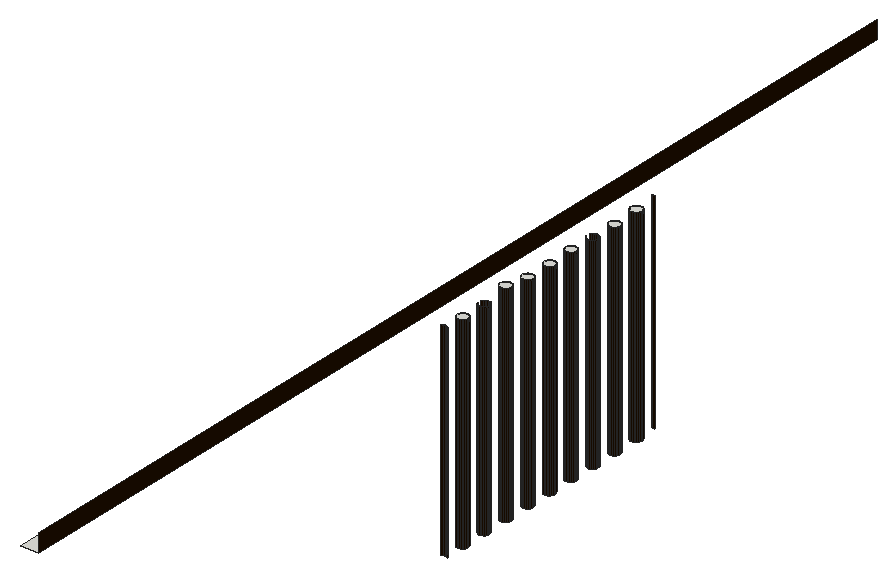
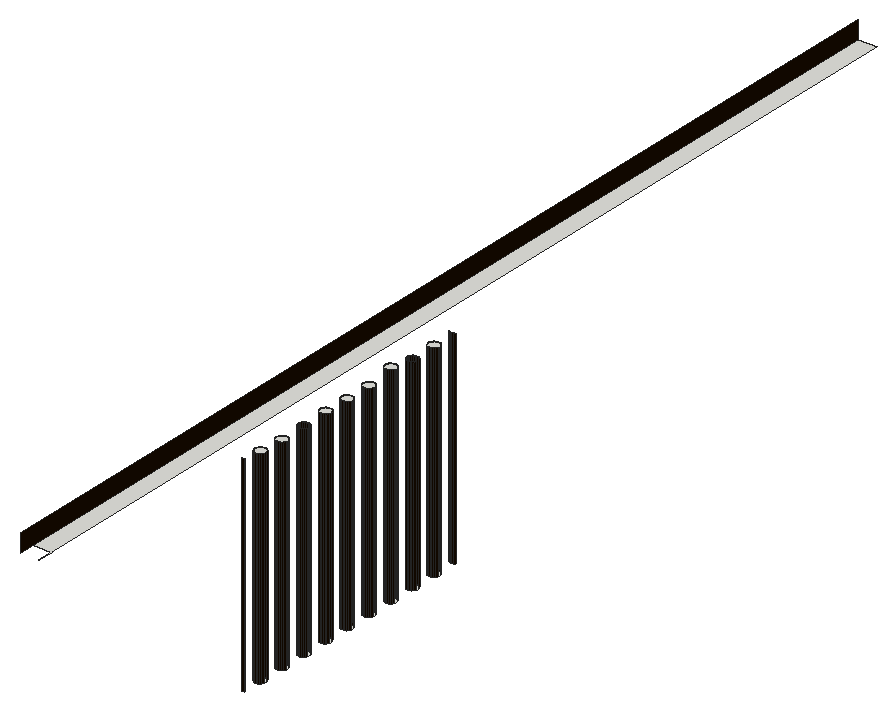
# SketchUp Ruby script. Lengths in inches.
U = 1.inch
M = Sketchup.active_model
def pt(a) = Geom::Point3d.new(a.map { |v| v * U })
def face(e, loops, mat)
  f = e.add_face(loops[0].map { |a| pt(a) })
  loops[1..].each { |l| e.add_face(l.map { |a| pt(a) }).erase! }
  f.material = f.back_material = mat if mat
  f
end
# faces: each face lists its corners as indices into pts; further lists are holes
def faces(e, pts, list, mat = nil) = list.each { |f| face(e, (f[0].is_a?(Array) ? f : [f]).map { |l| l.map { |i| pts[i] } }, mat) }
# xy, xz, yz: faces in a plane at the given z, y or x. An outline is a flat list of corners, or four numbers for a rectangle; further outlines are holes
def ring(l) = l.size == 4 ? [[l[0], l[1]], [l[2], l[1]], [l[2], l[3]], [l[0], l[3]]] : l.each_slice(2).to_a
def flat(e, list, mat, &to3) = list.each { |f| face(e, (f[0].is_a?(Array) ? f : [f]).map { |l| ring(l).map { |u, v| to3.(u, v) } }, mat) }
def xy(e, z, list, mat = nil) = flat(e, list, mat) { |x, y| [x, y, z] }
def xz(e, y, list, mat = nil) = flat(e, list, mat) { |x, z| [x, y, z] }
def yz(e, x, list, mat = nil) = flat(e, list, mat) { |y, z| [x, y, z] }
def lines(e, pts, list) = list.each { |a, b| e.add_line(pt(pts[a]), pt(pts[b])) }
# prism: a flat outline (further loops are holes) pulled along v
def prism(e, loops, v, mat = nil)
  f = face(e, loops, mat); d = Geom::Vector3d.new(v.map { |x| x * U })
  f.pushpull(f.normal.samedirection?(d) ? d.length : -d.length)
end
def box(e, o, s, mat = nil) = prism(e, [[o, [o[0] + s[0], o[1], o[2]], [o[0] + s[0], o[1] + s[1], o[2]], [o[0], o[1] + s[1], o[2]]]], [0, 0, s[2]], mat)
def at(x, y, z, deg = 0) = Geom::Transformation.translation(pt([x, y, z])) * Geom::Transformation.rotation(ORIGIN, Z_AXIS, deg.degrees)
def axes(o, x, y, z) = Geom::Transformation.new([*x, 0, *y, 0, *z, 0, *pt(o).to_a, 1])
def part(name) = M.definitions.add(name)
# library, detail: a bought-in or finely detailed component or shape, given as its bounding box
def library(name, o, s) = part(name).tap { |d| box(d.entities, o, s) }
def detail(e, o, s) = box(e.add_group.entities, o, s)
def put(e, d, t, mat = nil) = e.add_instance(d, t).tap { |i| i.material = mat if mat }
def group(e, t, mat = nil) = e.add_group.tap { |g| g.transformation = t; g.material = mat if mat }.entities
root = M.entities
M.materials.add("[Metal Seamed]1").color = [28, 14, 0]
xy(root,618.25,[[363.55,200.72,363.21,200.81,362.92,200.98,362.67,201.22,362.5,201.52,362.41,201.85,362.41,202.19,362.5,202.52,362.67,202.82,362.91,203.0625,363.2,203.24,363.54,203.33,363.88,203.33,364.21,203.24,364.51,203.07,364.75,202.83,364.92,202.53,365.01,202.2,365.01,201.86,364.93,201.53,364.76,201.23,364.51,200.99,364.22,200.8125,363.89,200.72],[363.55,207.16,363.21,207.25,362.92,207.42,362.67,207.66,362.5,207.96,362.41,208.29,362.41,208.63,362.5,208.96,362.67,209.26,362.91,209.5,363.2,209.67,363.54,209.76,363.88,209.76,364.21,209.68,364.51,209.51,364.75,209.26,364.92,208.97,365.01,208.64,365.01,208.3,364.93,207.96,364.76,207.67,364.51,207.42,364.22,207.25,363.89,207.16],[363.55,213.6,363.21,213.69,362.92,213.86,362.67,214.1,362.5,214.39,362.41,214.72,362.41,215.07,362.5,215.4,362.67,215.69,362.91,215.9375,363.2,216.11,363.54,216.2,363.88,216.2,364.21,216.11,364.51,215.94,364.75,215.7,364.92,215.41,365.01,215.08,365.01,214.73,364.93,214.4,364.76,214.1,364.51,213.86,364.22,213.6875,363.89,213.6],[363.55,220.04,363.21,220.12,362.92,220.29,362.67,220.53,362.5,220.83,362.41,221.16,362.41,221.5,362.5,221.83,362.67,222.13,362.91,222.375,363.2,222.55,363.54,222.64,363.88,222.64,364.21,222.55,364.51,222.38,364.75,222.14,364.92,221.84,365.01,221.51,365.01,221.17,364.93,220.84,364.76,220.54,364.51,220.3,364.22,220.125,363.89,220.04],[363.55,226.47,363.21,226.56,362.92,226.73,362.67,226.97,362.5,227.27,362.41,227.6,362.41,227.94,362.5,228.27,362.67,228.57,362.91,228.8125,363.2,228.99,363.54,229.08,363.88,229.08,364.21,228.99,364.51,228.82,364.75,228.58,364.92,228.28,365.01,227.95,365.01,227.61,364.93,227.28,364.76,226.98,364.51,226.74,364.22,226.5625,363.89,226.47],
  [363.55,232.91,363.21,233,362.92,233.17,362.67,233.41,362.5,233.71,362.41,234.04,362.41,234.38,362.5,234.71,362.67,235.01,362.91,235.25,363.2,235.42,363.54,235.51,363.88,235.51,364.21,235.43,364.51,235.26,364.75,235.01,364.92,234.72,365.01,234.39,365.01,234.05,364.93,233.71,364.76,233.42,364.51,233.17,364.22,233,363.89,232.91],[363.55,239.35,363.21,239.44,362.92,239.61,362.67,239.85,362.5,240.14,362.41,240.47,362.41,240.82,362.5,241.15,362.67,241.44,362.91,241.6875,363.2,241.86,363.54,241.95,363.88,241.95,364.21,241.86,364.51,241.69,364.75,241.45,364.92,241.16,365.01,240.83,365.01,240.48,364.93,240.15,364.76,239.85,364.51,239.61,364.22,239.4375,363.89,239.35],[363.55,245.79,363.21,245.87,362.92,246.04,362.67,246.28,362.5,246.58,362.41,246.91,362.41,247.25,362.5,247.58,362.67,247.88,362.91,248.125,363.2,248.3,363.54,248.39,363.88,248.39,364.21,248.3,364.51,248.13,364.75,247.89,364.92,247.59,365.01,247.26,365.01,246.92,364.93,246.59,364.76,246.29,364.51,246.05,364.22,245.875,363.89,245.79],[363.55,252.22,363.21,252.31,362.92,252.48,362.67,252.72,362.5,253.02,362.41,253.35,362.41,253.69,362.5,254.02,362.67,254.32,362.91,254.5625,363.2,254.74,363.54,254.83,363.88,254.83,364.21,254.74,364.51,254.57,364.75,254.33,364.92,254.03,365.01,253.7,365.01,253.36,364.93,253.03,364.76,252.73,364.51,252.49,364.22,252.3125,363.89,252.22]])
xy(root,666.625,[[363.55,245.79,363.89,245.79,364.22,245.875,364.51,246.05,364.76,246.29,364.93,246.59,365.01,246.92,365.01,247.26,364.92,247.59,364.75,247.89,364.51,248.13,364.21,248.3,363.88,248.39,363.54,248.39,363.2,248.3,362.91,248.125,362.67,247.88,362.5,247.58,362.41,247.25,362.41,246.91,362.5,246.58,362.67,246.28,362.92,246.04,363.21,245.87]])
xy(root,666.75,[[363.55,220.04,363.89,220.04,364.22,220.125,364.51,220.3,364.76,220.54,364.93,220.84,365.01,221.17,365.01,221.51,364.92,221.84,364.75,222.14,364.51,222.38,364.21,222.55,363.88,222.64,363.54,222.64,363.2,222.55,362.91,222.375,362.67,222.13,362.5,221.83,362.41,221.5,362.41,221.16,362.5,220.83,362.67,220.53,362.92,220.29,363.21,220.12],[363.55,226.47,363.89,226.47,364.22,226.5625,364.51,226.74,364.76,226.98,364.93,227.28,365.01,227.61,365.01,227.95,364.92,228.28,364.75,228.58,364.51,228.82,364.21,228.99,363.88,229.08,363.54,229.08,363.2,228.99,362.91,228.8125,362.67,228.57,362.5,228.27,362.41,227.94,362.41,227.6,362.5,227.27,362.67,226.97,362.92,226.73,363.21,226.56]])
xy(root,666.8125,[[363.55,200.72,363.89,200.72,364.22,200.8125,364.51,200.99,364.76,201.23,364.93,201.53,365.01,201.86,365.01,202.2,364.92,202.53,364.75,202.83,364.51,203.07,364.21,203.24,363.88,203.33,363.54,203.33,363.2,203.24,362.91,203.0625,362.67,202.82,362.5,202.52,362.41,202.19,362.41,201.85,362.5,201.52,362.67,201.22,362.92,200.98,363.21,200.81]])
xy(root,666.9375,[[363.55,232.91,363.89,232.91,364.22,233,364.51,233.17,364.76,233.42,364.93,233.71,365.01,234.05,365.01,234.39,364.92,234.72,364.75,235.01,364.51,235.26,364.21,235.43,363.88,235.51,363.54,235.51,363.2,235.42,362.91,235.25,362.67,235.01,362.5,234.71,362.41,234.38,362.41,234.04,362.5,233.71,362.67,233.41,362.92,233.17,363.21,233]])
xy(root,667,[[363.55,252.22,363.89,252.22,364.22,252.3125,364.51,252.49,364.76,252.73,364.93,253.03,365.01,253.36,365.01,253.7,364.92,254.03,364.75,254.33,364.51,254.57,364.21,254.74,363.88,254.83,363.54,254.83,363.2,254.74,362.91,254.5625,362.67,254.32,362.5,254.02,362.41,253.69,362.41,253.35,362.5,253.02,362.67,252.72,362.92,252.48,363.21,252.31]])
xy(root,667.8125,[[363.55,213.6,363.89,213.6,364.22,213.6875,364.51,213.86,364.76,214.1,364.93,214.4,365.01,214.73,365.01,215.08,364.92,215.41,364.75,215.7,364.51,215.94,364.21,216.11,363.88,216.2,363.54,216.2,363.2,216.11,362.91,215.9375,362.67,215.69,362.5,215.4,362.41,215.07,362.41,214.72,362.5,214.39,362.67,214.1,362.92,213.86,363.21,213.69]])
xy(root,674.05,[[361.97,73.28,361.97,321.28,361.98,321.28,361.98,317.52,366.34,317.52,366.34,73.28]])
xz(root,196.89,[[363.54,618.25,363.88,667.125]],"[Metal Seamed]1")
xz(root,200.72,[[363.55,618.25,363.89,666.8125]],"[Metal Seamed]1")
xz(root,203.33,[[363.54,618.25,363.88,666.8125]],"[Metal Seamed]1")
xz(root,207.16,[[363.55,618.25,363.89,666.66]],"[Metal Seamed]1")
xz(root,209.76,[[363.54,618.25,363.88,666.66]],"[Metal Seamed]1")
xz(root,213.6,[[363.55,618.25,363.89,667.8125]],"[Metal Seamed]1")
xz(root,216.2,[[363.54,618.25,363.88,667.8125]],"[Metal Seamed]1")
xz(root,220.04,[[363.55,618.25,363.89,666.75]],"[Metal Seamed]1")
xz(root,222.64,[[363.54,618.25,363.88,666.75]],"[Metal Seamed]1")
xz(root,226.47,[[363.55,618.25,363.89,666.75]],"[Metal Seamed]1")
xz(root,229.08,[[363.54,618.25,363.88,666.75]],"[Metal Seamed]1")
xz(root,232.91,[[363.55,618.25,363.89,666.9375]],"[Metal Seamed]1")
xz(root,235.51,[[363.54,618.25,363.88,666.9375]],"[Metal Seamed]1")
xz(root,239.35,[[363.55,618.25,363.89,666.66]],"[Metal Seamed]1")
xz(root,241.95,[[363.54,618.25,363.88,666.66]],"[Metal Seamed]1")
xz(root,245.79,[[363.55,618.25,363.89,666.625]],"[Metal Seamed]1")
xz(root,248.39,[[363.54,618.25,363.88,666.625]],"[Metal Seamed]1")
xz(root,252.22,[[363.55,618.25,363.89,667]],"[Metal Seamed]1")
xz(root,254.83,[[363.54,618.25,363.88,667]],"[Metal Seamed]1")
xz(root,258.66,[[363.55,618.25,363.89,667.625]],"[Metal Seamed]1")
yz(root,365.01,[[201.86,618.25,202.2,666.8125],[208.3,618.25,208.64,666.66],[214.73,618.25,215.08,667.8125],[221.17,618.25,221.51,666.75],[227.61,618.25,227.95,666.75],
  [234.05,618.25,234.39,666.9375],[240.48,618.25,240.83,666.66],[246.92,618.25,247.26,666.625],[253.36,618.25,253.7,667]],"[Metal Seamed]1")
yz(root,366.34,[[73.28,674.05,321.28,678.3125]],"[Metal Seamed]1")
p = [[363.2,196.8,618.25],[362.91,196.625,618.25],[362.91,196.625,667.125],[363.2,196.8,667.125],[364.51,196.63,618.25],[364.21,196.8,618.25],
  [364.21,196.8,667.125],[364.51,196.63,667.125],[363.54,196.89,618.25],[363.54,196.89,667.125],[363.88,196.89,618.25],[363.88,196.89,667.125],
  [363.21,200.81,618.25],[363.55,200.72,618.25],[363.55,200.72,666.8125],[363.21,200.81,666.8125],[363.89,200.72,618.25],[364.22,200.8125,618.25],
  [364.22,200.8125,666.8125],[363.89,200.72,666.8125],[362.92,200.98,618.25],[362.92,200.98,666.8125],[364.51,200.99,618.25],[364.51,200.99,666.8125],
  [362.67,201.22,618.25],[362.67,201.22,666.8125],[364.76,201.23,618.25],[364.76,201.23,666.8125],[362.5,201.52,618.25],[362.5,201.52,666.8125],
  [364.93,201.53,618.25],[364.93,201.53,666.8125],[365.01,201.86,618.25],[365.01,201.86,666.8125],[365.01,202.2,618.25],[364.92,202.53,618.25],
  [364.92,202.53,666.8125],[365.01,202.2,666.8125],[362.67,202.82,618.25],[362.5,202.52,618.25],[362.5,202.52,666.8125],[362.67,202.82,666.8125],
  [364.75,202.83,618.25],[364.75,202.83,666.8125],[362.91,203.0625,618.25],[362.91,203.0625,666.8125],[364.51,203.07,618.25],[364.51,203.07,666.8125],
  [363.2,203.24,618.25],[363.2,203.24,666.8125],[364.21,203.24,618.25],[364.21,203.24,666.8125],[363.54,203.33,618.25],[363.54,203.33,666.8125],
  [363.88,203.33,618.25],[363.88,203.33,666.8125],[362.92,207.42,618.25],[363.21,207.25,618.25],[363.21,207.25,666.66],[362.92,207.42,666.66],
  [363.55,207.16,618.25],[363.55,207.16,666.66],[363.89,207.16,618.25],[364.22,207.25,618.25],[364.22,207.25,666.66],[363.89,207.16,666.66],
  [364.51,207.42,618.25],[364.51,207.42,666.66],[362.67,207.66,618.25],[362.67,207.66,666.66],[364.76,207.67,618.25],[364.76,207.67,666.66],
  [362.5,207.96,618.25],[362.5,207.96,666.66],[364.93,207.96,618.25],[364.93,207.96,666.66],[365.01,208.3,618.25],[365.01,208.3,666.66],
  [365.01,208.64,618.25],[364.92,208.97,618.25],[364.92,208.97,666.66],[365.01,208.64,666.66],[362.67,209.26,618.25],[362.5,208.96,618.25],
  [362.5,208.96,666.66],[362.67,209.26,666.66],[364.75,209.26,618.25],[364.75,209.26,666.66],[362.91,209.5,618.25],[362.91,209.5,666.66],
  [364.51,209.51,618.25],[364.51,209.51,666.66],[363.2,209.67,618.25],[363.2,209.67,666.66],[364.21,209.68,618.25],[364.21,209.68,666.66],
  [363.54,209.76,618.25],[363.54,209.76,666.66],[363.88,209.76,618.25],[363.88,209.76,666.66],[363.21,213.69,618.25],[363.55,213.6,618.25],
  [363.55,213.6,667.8125],[363.21,213.69,667.8125],[363.89,213.6,618.25],[364.22,213.6875,618.25],[364.22,213.6875,667.8125],[363.89,213.6,667.8125],
  [362.92,213.86,618.25],[362.92,213.86,667.8125],[364.51,213.86,618.25],[364.51,213.86,667.8125],[362.67,214.1,618.25],[362.67,214.1,667.8125],
  [364.76,214.1,618.25],[364.76,214.1,667.8125],[362.5,214.39,618.25],[362.5,214.39,667.8125],[364.93,214.4,618.25],[364.93,214.4,667.8125],
  [365.01,214.73,618.25],[365.01,214.73,667.8125],[365.01,215.08,618.25],[364.92,215.41,618.25],[364.92,215.41,667.8125],[365.01,215.08,667.8125],
  [362.67,215.69,618.25],[362.5,215.4,618.25],[362.5,215.4,667.8125],[362.67,215.69,667.8125],[364.75,215.7,618.25],[364.75,215.7,667.8125],
  [362.91,215.9375,618.25],[362.91,215.9375,667.8125],[364.51,215.94,618.25],[364.51,215.94,667.8125],[363.2,216.11,618.25],[363.2,216.11,667.8125],
  [364.21,216.11,618.25],[364.21,216.11,667.8125],[363.54,216.2,618.25],[363.54,216.2,667.8125],[363.88,216.2,618.25],[363.88,216.2,667.8125],
  [363.21,220.12,618.25],[363.55,220.04,618.25],[363.55,220.04,666.75],[363.21,220.12,666.75],[363.89,220.04,618.25],[364.22,220.125,618.25],
  [364.22,220.125,666.75],[363.89,220.04,666.75],[362.92,220.29,618.25],[362.92,220.29,666.75],[364.51,220.3,618.25],[364.51,220.3,666.75],
  [362.67,220.53,618.25],[362.67,220.53,666.75],[364.76,220.54,618.25],[364.76,220.54,666.75],[362.5,220.83,618.25],[362.5,220.83,666.75],
  [364.93,220.84,618.25],[364.93,220.84,666.75],[365.01,221.17,618.25],[365.01,221.17,666.75],[365.01,221.51,618.25],[364.92,221.84,618.25],
  [364.92,221.84,666.75],[365.01,221.51,666.75],[362.67,222.13,618.25],[362.5,221.83,618.25],[362.5,221.83,666.75],[362.67,222.13,666.75],
  [364.75,222.14,618.25],[364.75,222.14,666.75],[362.91,222.375,618.25],[362.91,222.375,666.75],[364.51,222.38,618.25],[364.51,222.38,666.75],
  [363.2,222.55,618.25],[363.2,222.55,666.75],[364.21,222.55,618.25],[364.21,222.55,666.75],[363.54,222.64,618.25],[363.54,222.64,666.75],
  [363.88,222.64,618.25],[363.88,222.64,666.75],[363.21,226.56,618.25],[363.55,226.47,618.25],[363.55,226.47,666.75],[363.21,226.56,666.75],
  [363.89,226.47,618.25],[364.22,226.5625,618.25],[364.22,226.5625,666.75],[363.89,226.47,666.75],[362.92,226.73,618.25],[362.92,226.73,666.75],
  [364.51,226.74,618.25],[364.51,226.74,666.75],[362.67,226.97,618.25],[362.67,226.97,666.75],[364.76,226.98,618.25],[364.76,226.98,666.75],
  [362.5,227.27,618.25],[362.5,227.27,666.75],[364.93,227.28,618.25],[364.93,227.28,666.75],[365.01,227.61,618.25],[365.01,227.61,666.75],
  [365.01,227.95,618.25],[364.92,228.28,618.25],[364.92,228.28,666.75],[365.01,227.95,666.75],[362.67,228.57,618.25],[362.5,228.27,618.25],
  [362.5,228.27,666.75],[362.67,228.57,666.75],[364.75,228.58,618.25],[364.75,228.58,666.75],[362.91,228.8125,618.25],[362.91,228.8125,666.75],
  [364.51,228.82,618.25],[364.51,228.82,666.75],[363.2,228.99,618.25],[363.2,228.99,666.75],[364.21,228.99,618.25],[364.21,228.99,666.75],
  [363.54,229.08,618.25],[363.54,229.08,666.75],[363.88,229.08,618.25],[363.88,229.08,666.75],[363.21,233,618.25],[363.55,232.91,618.25],
  [363.55,232.91,666.9375],[363.21,233,666.9375],[363.89,232.91,618.25],[364.22,233,618.25],[364.22,233,666.9375],[363.89,232.91,666.9375],
  [362.92,233.17,618.25],[362.92,233.17,666.9375],[364.51,233.17,618.25],[364.51,233.17,666.9375],[362.67,233.41,618.25],[362.67,233.41,666.9375],
  [364.76,233.42,618.25],[364.76,233.42,666.9375],[362.5,233.71,618.25],[362.5,233.71,666.9375],[364.93,233.71,618.25],[364.93,233.71,666.9375],
  [365.01,234.05,618.25],[365.01,234.05,666.9375],[365.01,234.39,618.25],[364.92,234.72,618.25],[364.92,234.72,666.9375],[365.01,234.39,666.9375],
  [362.67,235.01,618.25],[362.5,234.71,618.25],[362.5,234.71,666.9375],[362.67,235.01,666.9375],[364.75,235.01,618.25],[364.75,235.01,666.9375],
  [362.91,235.25,618.25],[362.91,235.25,666.9375],[364.51,235.26,618.25],[364.51,235.26,666.9375],[363.2,235.42,618.25],[363.2,235.42,666.9375],
  [364.21,235.43,618.25],[364.21,235.43,666.9375],[363.54,235.51,618.25],[363.54,235.51,666.9375],[363.88,235.51,618.25],[363.88,235.51,666.9375],
  [363.21,239.44,618.25],[363.55,239.35,618.25],[363.55,239.35,666.66],[363.21,239.44,666.66],[363.89,239.35,618.25],[364.22,239.4375,618.25],
  [364.22,239.4375,666.66],[363.89,239.35,666.66],[362.92,239.61,618.25],[362.92,239.61,666.66],[364.51,239.61,618.25],[364.51,239.61,666.66],
  [362.67,239.85,618.25],[362.67,239.85,666.66],[364.76,239.85,618.25],[364.76,239.85,666.66],[362.5,240.14,618.25],[362.5,240.14,666.66],
  [364.93,240.15,618.25],[364.93,240.15,666.66],[365.01,240.48,618.25],[365.01,240.48,666.66],[365.01,240.83,618.25],[364.92,241.16,618.25],
  [364.92,241.16,666.66],[365.01,240.83,666.66],[362.67,241.44,618.25],[362.5,241.15,618.25],[362.5,241.15,666.66],[362.67,241.44,666.66],
  [364.75,241.45,618.25],[364.75,241.45,666.66],[362.91,241.6875,618.25],[362.91,241.6875,666.66],[364.51,241.69,618.25],[364.51,241.69,666.66],
  [363.2,241.86,618.25],[363.2,241.86,666.66],[364.21,241.86,618.25],[364.21,241.86,666.66],[363.54,241.95,618.25],[363.54,241.95,666.66],
  [363.88,241.95,618.25],[363.88,241.95,666.66],[363.21,245.87,618.25],[363.55,245.79,618.25],[363.55,245.79,666.625],[363.21,245.87,666.625],
  [363.89,245.79,618.25],[364.22,245.875,618.25],[364.22,245.875,666.625],[363.89,245.79,666.625],[362.92,246.04,618.25],[362.92,246.04,666.625],
  [364.51,246.05,618.25],[364.51,246.05,666.625],[362.67,246.28,618.25],[362.67,246.28,666.625],[364.76,246.29,618.25],[364.76,246.29,666.625],
  [362.5,246.58,618.25],[362.5,246.58,666.625],[364.93,246.59,618.25],[364.93,246.59,666.625],[365.01,246.92,618.25],[365.01,246.92,666.625],
  [365.01,247.26,618.25],[364.92,247.59,618.25],[364.92,247.59,666.625],[365.01,247.26,666.625],[362.67,247.88,618.25],[362.5,247.58,618.25],
  [362.5,247.58,666.625],[362.67,247.88,666.625],[364.75,247.89,618.25],[364.75,247.89,666.625],[362.91,248.125,618.25],[362.91,248.125,666.625],
  [364.51,248.13,618.25],[364.51,248.13,666.625],[363.2,248.3,618.25],[363.2,248.3,666.625],[364.21,248.3,618.25],[364.21,248.3,666.625],
  [363.54,248.39,618.25],[363.54,248.39,666.625],[363.88,248.39,618.25],[363.88,248.39,666.625],[363.21,252.31,618.25],[363.55,252.22,618.25],
  [363.55,252.22,667],[363.21,252.31,667],[363.89,252.22,618.25],[364.22,252.3125,618.25],[364.22,252.3125,667],[363.89,252.22,667],
  [362.92,252.48,618.25],[362.92,252.48,667],[364.51,252.49,618.25],[364.51,252.49,667],[362.67,252.72,618.25],[362.67,252.72,667],
  [364.76,252.73,618.25],[364.76,252.73,667],[362.5,253.02,618.25],[362.5,253.02,667],[364.93,253.03,618.25],[364.93,253.03,667],
  [365.01,253.36,618.25],[365.01,253.36,667],[365.01,253.7,618.25],[364.92,254.03,618.25],[364.92,254.03,667],[365.01,253.7,667],
  [362.67,254.32,618.25],[362.5,254.02,618.25],[362.5,254.02,667],[362.67,254.32,667],[364.75,254.33,618.25],[364.75,254.33,667],
  [362.91,254.5625,618.25],[362.91,254.5625,667],[364.51,254.57,618.25],[364.51,254.57,667],[363.2,254.74,618.25],[363.2,254.74,667],
  [364.21,254.74,618.25],[364.21,254.74,667],[363.54,254.83,618.25],[363.54,254.83,667],[363.88,254.83,618.25],[363.88,254.83,667],
  [363.21,258.75,618.25],[363.55,258.66,618.25],[363.55,258.66,667.625],[363.21,258.75,667.625]]
faces(root,p,[[0,1,2,3],[4,5,6,7],[8,0,3,9],[5,10,11,6],[12,13,14,15],[16,17,18,19],[20,12,15,21],[17,22,23,18],
  [24,20,21,25],[22,26,27,23],[28,24,25,29],[26,30,31,27],[30,32,33,31],[34,35,36,37],[38,39,40,41],[35,42,43,36],
  [44,38,41,45],[42,46,47,43],[48,44,45,49],[46,50,51,47],[52,48,49,53],[50,54,55,51],[56,57,58,59],[57,60,61,58],
  [62,63,64,65],[63,66,67,64],[68,56,59,69],[66,70,71,67],[72,68,69,73],[70,74,75,71],[74,76,77,75],[78,79,80,81],
  [82,83,84,85],[79,86,87,80],[88,82,85,89],[86,90,91,87],[92,88,89,93],[90,94,95,91],[96,92,93,97],[94,98,99,95],
  [100,101,102,103],[104,105,106,107],[108,100,103,109],[105,110,111,106],[112,108,109,113],[110,114,115,111],[116,112,113,117],[114,118,119,115],
  [118,120,121,119],[122,123,124,125],[126,127,128,129],[123,130,131,124],[132,126,129,133],[130,134,135,131],[136,132,133,137],[134,138,139,135],
  [140,136,137,141],[138,142,143,139],[144,145,146,147],[148,149,150,151],[152,144,147,153],[149,154,155,150],[156,152,153,157],[154,158,159,155],
  [160,156,157,161],[158,162,163,159],[162,164,165,163],[166,167,168,169],[170,171,172,173],[167,174,175,168],[176,170,173,177],[174,178,179,175],
  [180,176,177,181],[178,182,183,179],[184,180,181,185],[182,186,187,183],[188,189,190,191],[192,193,194,195],[196,188,191,197],[193,198,199,194],
  [200,196,197,201],[198,202,203,199],[204,200,201,205],[202,206,207,203],[206,208,209,207],[210,211,212,213],[214,215,216,217],[211,218,219,212],
  [220,214,217,221],[218,222,223,219],[224,220,221,225],[222,226,227,223],[228,224,225,229],[226,230,231,227],[232,233,234,235],[236,237,238,239],
  [240,232,235,241],[237,242,243,238],[244,240,241,245],[242,246,247,243],[248,244,245,249],[246,250,251,247],[250,252,253,251],[254,255,256,257],
  [258,259,260,261],[255,262,263,256],[264,258,261,265],[262,266,267,263],[268,264,265,269],[266,270,271,267],[272,268,269,273],[270,274,275,271],
  [276,277,278,279],[280,281,282,283],[284,276,279,285],[281,286,287,282],[288,284,285,289],[286,290,291,287],[292,288,289,293],[290,294,295,291],
  [294,296,297,295],[298,299,300,301],[302,303,304,305],[299,306,307,300],[308,302,305,309],[306,310,311,307],[312,308,309,313],[310,314,315,311],
  [316,312,313,317],[314,318,319,315],[320,321,322,323],[324,325,326,327],[328,320,323,329],[325,330,331,326],[332,328,329,333],[330,334,335,331],
  [336,332,333,337],[334,338,339,335],[338,340,341,339],[342,343,344,345],[346,347,348,349],[343,350,351,344],[352,346,349,353],[350,354,355,351],
  [356,352,353,357],[354,358,359,355],[360,356,357,361],[358,362,363,359],[364,365,366,367],[368,369,370,371],[372,364,367,373],[369,374,375,370],
  [376,372,373,377],[374,378,379,375],[380,376,377,381],[378,382,383,379],[382,384,385,383],[386,387,388,389],[390,391,392,393],[387,394,395,388],
  [396,390,393,397],[394,398,399,395],[400,396,397,401],[398,402,403,399],[404,400,401,405],[402,406,407,403],[408,409,410,411]],"[Metal Seamed]1")
